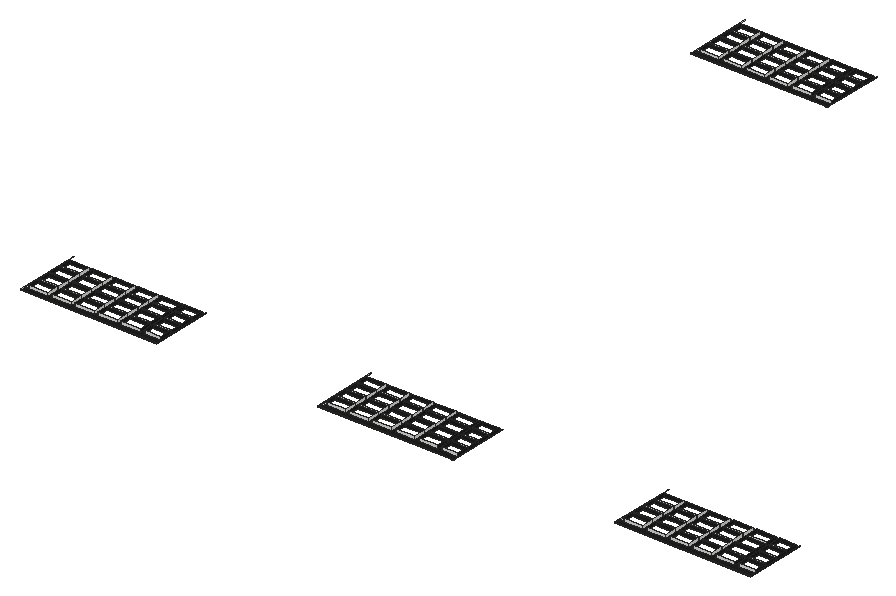
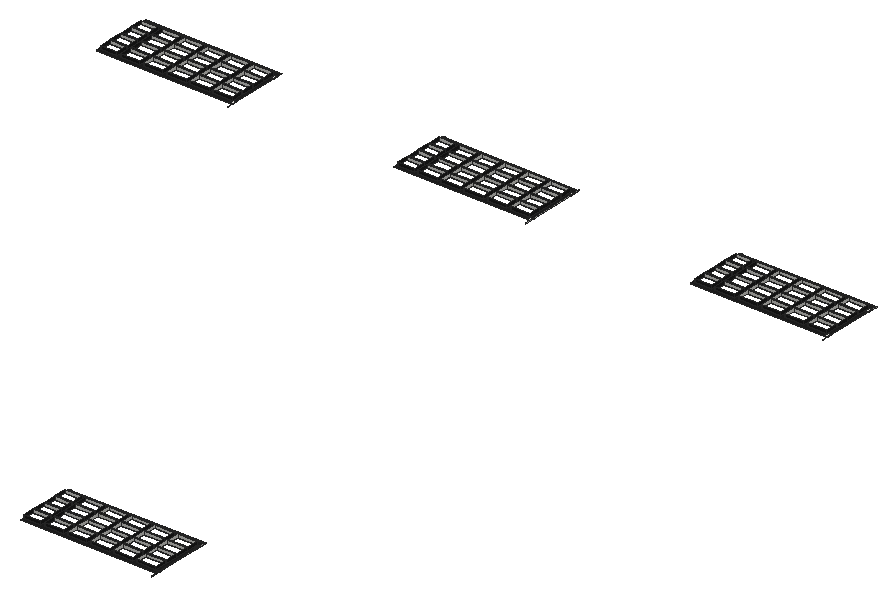
# SketchUp Ruby script. Lengths in inches.
U = 1.inch
M = Sketchup.active_model
def pt(a) = Geom::Point3d.new(a.map { |v| v * U })
def face(e, loops, mat)
  f = e.add_face(loops[0].map { |a| pt(a) })
  loops[1..].each { |l| e.add_face(l.map { |a| pt(a) }).erase! }
  f.material = f.back_material = mat if mat
  f
end
# faces: each face lists its corners as indices into pts; further lists are holes
def faces(e, pts, list, mat = nil) = list.each { |f| face(e, (f[0].is_a?(Array) ? f : [f]).map { |l| l.map { |i| pts[i] } }, mat) }
# xy, xz, yz: faces in a plane at the given z, y or x. An outline is a flat list of corners, or four numbers for a rectangle; further outlines are holes
def ring(l) = l.size == 4 ? [[l[0], l[1]], [l[2], l[1]], [l[2], l[3]], [l[0], l[3]]] : l.each_slice(2).to_a
def flat(e, list, mat, &to3) = list.each { |f| face(e, (f[0].is_a?(Array) ? f : [f]).map { |l| ring(l).map { |u, v| to3.(u, v) } }, mat) }
def xy(e, z, list, mat = nil) = flat(e, list, mat) { |x, y| [x, y, z] }
def xz(e, y, list, mat = nil) = flat(e, list, mat) { |x, z| [x, y, z] }
def yz(e, x, list, mat = nil) = flat(e, list, mat) { |y, z| [x, y, z] }
def lines(e, pts, list) = list.each { |a, b| e.add_line(pt(pts[a]), pt(pts[b])) }
# prism: a flat outline (further loops are holes) pulled along v
def prism(e, loops, v, mat = nil)
  f = face(e, loops, mat); d = Geom::Vector3d.new(v.map { |x| x * U })
  f.pushpull(f.normal.samedirection?(d) ? d.length : -d.length)
end
def box(e, o, s, mat = nil) = prism(e, [[o, [o[0] + s[0], o[1], o[2]], [o[0] + s[0], o[1] + s[1], o[2]], [o[0], o[1] + s[1], o[2]]]], [0, 0, s[2]], mat)
def at(x, y, z, deg = 0) = Geom::Transformation.translation(pt([x, y, z])) * Geom::Transformation.rotation(ORIGIN, Z_AXIS, deg.degrees)
def axes(o, x, y, z) = Geom::Transformation.new([*x, 0, *y, 0, *z, 0, *pt(o).to_a, 1])
def part(name) = M.definitions.add(name)
# library, detail: a bought-in or finely detailed component or shape, given as its bounding box
def library(name, o, s) = part(name).tap { |d| box(d.entities, o, s) }
def detail(e, o, s) = box(e.add_group.entities, o, s)
def put(e, d, t, mat = nil) = e.add_instance(d, t).tap { |i| i.material = mat if mat }
def group(e, t, mat = nil) = e.add_group.tap { |g| g.transformation = t; g.material = mat if mat }.entities
root = M.entities
M.materials.add("[Color M08]").color = [30, 30, 30]
xy(root,115.91,[[264.14,322.4375,270.875,322.71],[1150.61,322.4375,1157.34,322.71],[2037.07,322.4375,2043.8,322.71],[264.14,322.71,270.875,334.4375],[1150.61,322.71,1157.34,334.4375],
  [2037.07,322.71,2043.8,334.4375],[264.14,475.3125,270.875,487.3125],[1150.61,475.3125,1157.34,487.3125],[2037.07,475.3125,2043.8,487.3125],[782.875,2174.43,789.61,2174.7],
  [782.875,2174.7,789.61,2186.43],[782.875,2327.31,789.61,2339.31]])
xy(root,115.91,[[[264.14,305.5,264.14,322.4375,270.875,322.4375,270.875,322.71,275.2,322.71,275.2,334.54,264.14,334.54,264.14,475.3125,275.36,475.3125,275.36,487.3125,671.22,487.3125,671.22,305.5],[412.875,323.5,470.84,323.5,470.84,356.95,412.875,356.95,412.875,362.375,470.84,362.375,470.84,396.41,412.875,396.41,412.875,401.625,470.84,401.625,470.84,435.86,412.875,435.86,412.875,441.875,470.84,441.875,470.84,475.3125,412.875,475.3125,412.875,435.86,401.9375,435.86,401.9375,475.3125,343.98,475.3125,343.98,401.625,401.9375,401.625,401.9375,396.41,343.98,396.41,343.98,362.375,401.9375,362.375,401.9375,435.86,412.875,435.86],[481.77,323.5,539.73,323.5,539.73,396.41,481.77,396.41,481.77,401.625,539.73,401.625,539.73,475.3125,481.77,475.3125,481.77,441.875,539.73,441.875,539.73,435.86,481.77,435.86],[550.67,323.5,608.63,435.86],[275.89,401.625,333.04,435.86],[275.89,362.375,333.04,396.41],[343.98,323.5,401.9375,356.95],[550.67,442.1875,608.63,475.3125],[275.89,323.5,333.04,356.95],[275.89,441.875,333.04,475.3125],[619.57,323.5,669.03,356.95],[619.57,362.95,669.03,396.41],[619.57,402.41,669.03,435.86],[619.57,441.86,669.03,475.3125]],[[1150.61,305.5,1150.61,322.4375,1157.34,322.4375,1157.34,322.71,1161.66,322.71,1161.66,334.54,1150.61,334.54,1150.61,475.3125,1161.82,475.3125,1161.82,487.3125,1557.68,487.3125,1557.68,305.5],[1299.34,323.5,1357.3,323.5,1357.3,356.95,1299.34,356.95,1299.34,362.375,1357.3,362.375,1357.3,396.41,1299.34,396.41,1299.34,401.625,1357.3,401.625,1357.3,435.86,1299.34,435.86,1299.34,441.875,1357.3,441.875,1357.3,475.3125,1299.34,475.3125,1299.34,435.86,1288.4,435.86,1288.4,475.3125,1230.44,475.3125,1230.44,401.625,1288.4,401.625,1288.4,396.41,1230.44,396.41,1230.44,362.375,1288.4,362.375,1288.4,435.86,1299.34,435.86],[1368.24,323.5,1426.2,323.5,1426.2,396.41,1368.24,396.41,1368.24,401.625,1426.2,401.625,1426.2,475.3125,1368.24,475.3125,1368.24,441.875,1426.2,441.875,1426.2,435.86,1368.24,435.86],[1437.14,323.5,1495.1,435.86],[1162.36,401.625,1219.5,435.86],[1162.36,362.375,1219.5,396.41],[1230.44,323.5,1288.4,356.95],[1437.14,442.1875,1495.1,475.3125],[1162.36,323.5,1219.5,356.95],[1162.36,441.875,1219.5,475.3125],[1506.03,323.5,1555.49,356.95],[1506.03,362.95,1555.49,396.41],[1506.03,402.41,1555.49,435.86],[1506.03,441.86,1555.49,475.3125]],[[2037.07,305.5,2037.07,322.4375,2043.8,322.4375,2043.8,322.71,2048.125,322.71,2048.125,334.54,2037.07,334.54,2037.07,475.3125,2048.29,475.3125,2048.29,487.3125,2444.15,487.3125,2444.15,305.5],[2185.8,323.5,2243.76,323.5,2243.76,356.95,2185.8,356.95,2185.8,362.375,2243.76,362.375,2243.76,396.41,2185.8,396.41,2185.8,401.625,2243.76,401.625,2243.76,435.86,2185.8,435.86,2185.8,441.875,2243.76,441.875,2243.76,475.3125,2185.8,475.3125,2185.8,435.86,2174.87,435.86,2174.87,475.3125,2116.91,475.3125,2116.91,401.625,2174.87,401.625,2174.87,396.41,2116.91,396.41,2116.91,362.375,2174.87,362.375,2174.87,435.86,2185.8,435.86],[2254.7,323.5,2312.66,323.5,2312.66,396.41,2254.7,396.41,2254.7,401.625,2312.66,401.625,2312.66,475.3125,2254.7,475.3125,2254.7,441.875,2312.66,441.875,2312.66,435.86,2254.7,435.86],[2323.6,323.5,2381.56,435.86],[2048.82,401.625,2105.97,435.86],[2048.82,362.375,2105.97,396.41],[2116.91,323.5,2174.87,356.95],[2323.6,442.1875,2381.56,475.3125],[2048.82,323.5,2105.97,356.95],[2048.82,441.875,2105.97,475.3125],[2392.5,323.5,2441.96,356.95],[2392.5,362.95,2441.96,396.41],[2392.5,402.41,2441.96,435.86],[2392.5,441.86,2441.96,475.3125]],[270.875,322.71,270.875,334.4375,264.14,334.4375,264.14,334.54,275.2,334.54,275.2,322.71],[1157.34,322.71,1157.34,334.4375,1150.61,334.4375,1150.61,334.54,1161.66,334.54,1161.66,322.71],
  [2043.8,322.71,2043.8,334.4375,2037.07,334.4375,2037.07,334.54,2048.125,334.54,2048.125,322.71],[481.77,356.95,539.73,362.375],[550.67,356.95,608.63,362.875],[1368.24,356.95,1426.2,362.375],[1437.14,356.95,1495.1,362.875],
  [2254.7,356.95,2312.66,362.375],[2323.6,356.95,2381.56,362.875],[550.67,396.41,608.63,401.75],[1437.14,396.41,1495.1,401.75],[2323.6,396.41,2381.56,401.75],
  [343.98,435.86,401.9375,441.875],[1230.44,435.86,1288.4,441.875],[2116.91,435.86,2174.87,441.875],[270.875,475.3125,275.36,487.3125],[1157.34,475.3125,1161.82,487.3125],
  [2043.8,475.3125,2048.29,487.3125],[[782.875,2157.49,782.875,2174.43,789.61,2174.43,789.61,2174.7,793.93,2174.7,793.93,2186.53,782.875,2186.53,782.875,2327.31,794.09,2327.31,794.09,2339.31,1189.95,2339.31,1189.95,2157.49],[931.61,2175.49,989.57,2175.49,989.57,2208.95,931.61,2208.95,931.61,2214.37,989.57,2214.37,989.57,2248.4,931.61,2248.4,931.61,2253.62,989.57,2253.62,989.57,2287.85,931.61,2287.85,931.61,2293.87,989.57,2293.87,989.57,2327.31,931.61,2327.31,931.61,2287.85,920.67,2287.85,920.67,2327.31,862.71,2327.31,862.71,2253.62,920.67,2253.62,920.67,2248.4,862.71,2248.4,862.71,2214.37,920.67,2214.37,920.67,2287.85,931.61,2287.85],[1000.51,2175.49,1058.47,2175.49,1058.47,2248.4,1000.51,2248.4,1000.51,2253.62,1058.47,2253.62,1058.47,2327.31,1000.51,2327.31,1000.51,2293.87,1058.47,2293.87,1058.47,2287.85,1000.51,2287.85],[1069.4,2175.49,1127.36,2287.85],[794.625,2253.62,851.77,2287.85],[794.625,2214.37,851.77,2248.4],[862.71,2175.49,920.67,2208.95],[1069.4,2294.18,1127.36,2327.31],[794.625,2175.49,851.77,2208.95],[794.625,2293.87,851.77,2327.31],[1138.3,2293.85,1187.76,2327.31],[1138.3,2175.49,1187.76,2208.95],[1138.3,2214.95,1187.76,2248.4],[1138.3,2254.4,1187.76,2287.85]],[789.61,2174.7,789.61,2186.43,782.875,2186.43,782.875,2186.53,793.93,2186.53,793.93,2174.7],[1000.51,2208.95,1058.47,2214.37],[1069.4,2208.95,1127.36,2214.87],
  [1069.4,2248.4,1127.36,2253.74],[862.71,2287.85,920.67,2293.87],[789.61,2327.31,794.09,2339.31]],"[Color M08]")
xz(root,305.5,[[264.14,115.91,671.22,117.06],[1150.61,115.91,1557.68,117.06],[2037.07,115.91,2444.15,117.06]],"[Color M08]")
xz(root,323.5,[[275.89,115.91,333.04,125.0625],[343.98,115.91,401.9375,125.0625],[412.875,115.91,470.84,125.0625],[481.77,115.91,539.73,125.0625],[550.67,115.91,608.63,125.0625],
  [619.57,115.91,669.03,125.0625],[1162.36,115.91,1219.5,125.0625],[1230.44,115.91,1288.4,125.0625],[1299.34,115.91,1357.3,125.0625],[1368.24,115.91,1426.2,125.0625],
  [1437.14,115.91,1495.1,125.0625],[1506.03,115.91,1555.49,125.0625],[2048.82,115.91,2105.97,125.0625],[2116.91,115.91,2174.87,125.0625],[2185.8,115.91,2243.76,125.0625],
  [2254.7,115.91,2312.66,125.0625],[2323.6,115.91,2381.56,125.0625],[2392.5,115.91,2441.96,125.0625]])
xz(root,356.95,[[275.89,115.91,333.04,125.0625],[343.98,115.91,401.9375,125.0625],[412.875,115.91,470.84,125.0625],[481.77,115.91,539.73,125.0625],[550.67,115.91,608.63,125.0625],
  [619.57,115.91,669.03,125.0625],[1162.36,115.91,1219.5,125.0625],[1230.44,115.91,1288.4,125.0625],[1299.34,115.91,1357.3,125.0625],[1368.24,115.91,1426.2,125.0625],
  [1437.14,115.91,1495.1,125.0625],[1506.03,115.91,1555.49,125.0625],[2048.82,115.91,2105.97,125.0625],[2116.91,115.91,2174.87,125.0625],[2185.8,115.91,2243.76,125.0625],
  [2254.7,115.91,2312.66,125.0625],[2323.6,115.91,2381.56,125.0625],[2392.5,115.91,2441.96,125.0625]],"[Color M08]")
xz(root,362.375,[[275.89,115.91,333.04,125.0625],[343.98,115.91,401.9375,125.0625],[412.875,115.91,470.84,125.0625],[481.77,115.91,539.73,125.0625],[1162.36,115.91,1219.5,125.0625],
  [1230.44,115.91,1288.4,125.0625],[1299.34,115.91,1357.3,125.0625],[1368.24,115.91,1426.2,125.0625],[2048.82,115.91,2105.97,125.0625],[2116.91,115.91,2174.87,125.0625],
  [2185.8,115.91,2243.76,125.0625],[2254.7,115.91,2312.66,125.0625]])
xz(root,362.875,[[550.67,115.91,608.63,125.0625],[1437.14,115.91,1495.1,125.0625],[2323.6,115.91,2381.56,125.0625]])
xz(root,362.95,[[619.57,115.91,669.03,125.0625],[1506.03,115.91,1555.49,125.0625],[2392.5,115.91,2441.96,125.0625]])
xz(root,396.41,[[275.89,115.91,333.04,125.0625],[343.98,115.91,401.9375,125.0625],[412.875,115.91,470.84,125.0625],[481.77,115.91,539.73,125.0625],[550.67,115.91,608.63,125.0625],
  [619.57,115.91,669.03,125.0625],[1162.36,115.91,1219.5,125.0625],[1230.44,115.91,1288.4,125.0625],[1299.34,115.91,1357.3,125.0625],[1368.24,115.91,1426.2,125.0625],
  [1437.14,115.91,1495.1,125.0625],[1506.03,115.91,1555.49,125.0625],[2048.82,115.91,2105.97,125.0625],[2116.91,115.91,2174.87,125.0625],[2185.8,115.91,2243.76,125.0625],
  [2254.7,115.91,2312.66,125.0625],[2323.6,115.91,2381.56,125.0625],[2392.5,115.91,2441.96,125.0625]],"[Color M08]")
xz(root,401.625,[[275.89,115.91,333.04,125.0625],[343.98,115.91,401.9375,125.0625],[412.875,115.91,470.84,125.0625],[481.77,115.91,539.73,125.0625],[1162.36,115.91,1219.5,125.0625],
  [1230.44,115.91,1288.4,125.0625],[1299.34,115.91,1357.3,125.0625],[1368.24,115.91,1426.2,125.0625],[2048.82,115.91,2105.97,125.0625],[2116.91,115.91,2174.87,125.0625],
  [2185.8,115.91,2243.76,125.0625],[2254.7,115.91,2312.66,125.0625]])
xz(root,401.75,[[550.67,115.91,608.63,125.0625],[1437.14,115.91,1495.1,125.0625],[2323.6,115.91,2381.56,125.0625]])
xz(root,402.41,[[619.57,115.91,669.03,125.0625],[1506.03,115.91,1555.49,125.0625],[2392.5,115.91,2441.96,125.0625]])
xz(root,435.86,[[275.89,115.91,333.04,125.0625],[343.98,115.91,401.9375,125.0625],[412.875,115.91,470.84,125.0625],[481.77,115.91,539.73,125.0625],[550.67,115.91,608.63,125.0625],
  [619.57,115.91,669.03,125.0625],[1162.36,115.91,1219.5,125.0625],[1230.44,115.91,1288.4,125.0625],[1299.34,115.91,1357.3,125.0625],[1368.24,115.91,1426.2,125.0625],
  [1437.14,115.91,1495.1,125.0625],[1506.03,115.91,1555.49,125.0625],[2048.82,115.91,2105.97,125.0625],[2116.91,115.91,2174.87,125.0625],[2185.8,115.91,2243.76,125.0625],
  [2254.7,115.91,2312.66,125.0625],[2323.6,115.91,2381.56,125.0625],[2392.5,115.91,2441.96,125.0625]],"[Color M08]")
xz(root,441.86,[[619.57,115.91,669.03,125.0625],[1506.03,115.91,1555.49,125.0625],[2392.5,115.91,2441.96,125.0625]])
xz(root,441.875,[[275.89,115.91,333.04,125.0625],[343.98,115.91,401.9375,125.0625],[412.875,115.91,470.84,125.0625],[481.77,115.91,539.73,125.0625],[1162.36,115.91,1219.5,125.0625],
  [1230.44,115.91,1288.4,125.0625],[1299.34,115.91,1357.3,125.0625],[1368.24,115.91,1426.2,125.0625],[2048.82,115.91,2105.97,125.0625],[2116.91,115.91,2174.87,125.0625],
  [2185.8,115.91,2243.76,125.0625],[2254.7,115.91,2312.66,125.0625]])
xz(root,442.1875,[[550.67,115.91,608.63,125.0625],[1437.14,115.91,1495.1,125.0625],[2323.6,115.91,2381.56,125.0625]])
xz(root,475.3125,[[275.89,115.91,333.04,125.0625],[343.98,115.91,401.9375,125.0625],[412.875,115.91,470.84,125.0625],[481.77,115.91,539.73,125.0625],[550.67,115.91,608.63,125.0625],
  [619.57,115.91,669.03,125.0625],[1162.36,115.91,1219.5,125.0625],[1230.44,115.91,1288.4,125.0625],[1299.34,115.91,1357.3,125.0625],[1368.24,115.91,1426.2,125.0625],
  [1437.14,115.91,1495.1,125.0625],[1506.03,115.91,1555.49,125.0625],[2048.82,115.91,2105.97,125.0625],[2116.91,115.91,2174.87,125.0625],[2185.8,115.91,2243.76,125.0625],
  [2254.7,115.91,2312.66,125.0625],[2323.6,115.91,2381.56,125.0625],[2392.5,115.91,2441.96,125.0625]],"[Color M08]")
xz(root,2157.49,[[782.875,115.91,1189.95,117.06]],"[Color M08]")
xz(root,2175.49,[[794.625,115.91,851.77,125.0625],[862.71,115.91,920.67,125.0625],[931.61,115.91,989.57,125.0625],[1000.51,115.91,1058.47,125.0625],[1069.4,115.91,1127.36,125.0625],
  [1138.3,115.91,1187.76,125.0625]])
xz(root,2208.95,[[794.625,115.91,851.77,125.0625],[862.71,115.91,920.67,125.0625],[931.61,115.91,989.57,125.0625],[1000.51,115.91,1058.47,125.0625],[1069.4,115.91,1127.36,125.0625],
  [1138.3,115.91,1187.76,125.0625]],"[Color M08]")
xz(root,2214.37,[[794.625,115.91,851.77,125.0625],[862.71,115.91,920.67,125.0625],[931.61,115.91,989.57,125.0625],[1000.51,115.91,1058.47,125.0625]])
xz(root,2214.87,[[1069.4,115.91,1127.36,125.0625]])
xz(root,2214.95,[[1138.3,115.91,1187.76,125.0625]])
xz(root,2248.4,[[794.625,115.91,851.77,125.0625],[862.71,115.91,920.67,125.0625],[931.61,115.91,989.57,125.0625],[1000.51,115.91,1058.47,125.0625],[1069.4,115.91,1127.36,125.0625],
  [1138.3,115.91,1187.76,125.0625]],"[Color M08]")
xz(root,2253.62,[[794.625,115.91,851.77,125.0625],[862.71,115.91,920.67,125.0625],[931.61,115.91,989.57,125.0625],[1000.51,115.91,1058.47,125.0625]])
xz(root,2253.74,[[1069.4,115.91,1127.36,125.0625]])
xz(root,2254.4,[[1138.3,115.91,1187.76,125.0625]])
xz(root,2287.85,[[794.625,115.91,851.77,125.0625],[862.71,115.91,920.67,125.0625],[931.61,115.91,989.57,125.0625],[1000.51,115.91,1058.47,125.0625],[1069.4,115.91,1127.36,125.0625],
  [1138.3,115.91,1187.76,125.0625]],"[Color M08]")
xz(root,2293.85,[[1138.3,115.91,1187.76,125.0625]])
xz(root,2293.87,[[794.625,115.91,851.77,125.0625],[862.71,115.91,920.67,125.0625],[931.61,115.91,989.57,125.0625],[1000.51,115.91,1058.47,125.0625]])
xz(root,2294.18,[[1069.4,115.91,1127.36,125.0625]])
xz(root,2327.31,[[794.625,115.91,851.77,125.0625],[862.71,115.91,920.67,125.0625],[931.61,115.91,989.57,125.0625],[1000.51,115.91,1058.47,125.0625],[1069.4,115.91,1127.36,125.0625],
  [1138.3,115.91,1187.76,125.0625]],"[Color M08]")
yz(root,264.14,[[305.5,115.66,322.71,115.91],[322.71,115.66,334.4375,115.91],[334.4375,115.66,475.3125,115.91],[475.3125,115.66,487.3125,115.91],[305.5,115.91,305.5,117.06,306.625,117.06,306.625,117.65,505.3125,117.65,505.3125,115.91]])
yz(root,264.14,[[487.3125,115.66,505.3125,115.91]],"[Color M08]")
yz(root,275.89,[[323.5,115.91,356.95,125.0625],[362.375,115.91,396.41,125.0625],[401.625,115.91,435.86,125.0625],[441.875,115.91,475.3125,125.0625]],"[Color M08]")
yz(root,333.04,[[323.5,115.91,356.95,125.0625],[362.375,115.91,396.41,125.0625],[401.625,115.91,435.86,125.0625],[441.875,115.91,475.3125,125.0625]])
yz(root,343.98,[[323.5,115.91,356.95,125.0625],[362.375,115.91,396.41,125.0625],[401.625,115.91,435.86,125.0625],[441.875,115.91,475.3125,125.0625]],"[Color M08]")
yz(root,401.9375,[[323.5,115.91,356.95,125.0625],[362.375,115.91,396.41,125.0625],[401.625,115.91,435.86,125.0625],[441.875,115.91,475.3125,125.0625]])
yz(root,412.875,[[323.5,115.91,356.95,125.0625],[362.375,115.91,396.41,125.0625],[401.625,115.91,435.86,125.0625],[441.875,115.91,475.3125,125.0625]],"[Color M08]")
yz(root,470.84,[[323.5,115.91,356.95,125.0625],[362.375,115.91,396.41,125.0625],[401.625,115.91,435.86,125.0625],[441.875,115.91,475.3125,125.0625]])
yz(root,481.77,[[323.5,115.91,356.95,125.0625],[362.375,115.91,396.41,125.0625],[401.625,115.91,435.86,125.0625],[441.875,115.91,475.3125,125.0625]],"[Color M08]")
yz(root,539.73,[[323.5,115.91,356.95,125.0625],[362.375,115.91,396.41,125.0625],[401.625,115.91,435.86,125.0625],[441.875,115.91,475.3125,125.0625]])
yz(root,550.67,[[323.5,115.91,356.95,125.0625],[362.875,115.91,396.41,125.0625],[401.75,115.91,435.86,125.0625],[442.1875,115.91,475.3125,125.0625]],"[Color M08]")
yz(root,608.63,[[323.5,115.91,356.95,125.0625],[362.875,115.91,396.41,125.0625],[401.75,115.91,435.86,125.0625],[442.1875,115.91,475.3125,125.0625]],"[Color M08]")
yz(root,619.57,[[323.5,115.91,356.95,125.0625],[362.95,115.91,396.41,125.0625],[402.41,115.91,435.86,125.0625],[441.86,115.91,475.3125,125.0625]],"[Color M08]")
yz(root,669.03,[[323.5,115.91,356.95,125.0625],[362.95,115.91,396.41,125.0625],[402.41,115.91,435.86,125.0625],[441.86,115.91,475.3125,125.0625]],"[Color M08]")
yz(root,671.22,[[305.5,115.91,487.3125,117.06]],"[Color M08]")
yz(root,782.875,[[2157.49,115.66,2174.7,115.91],[2174.7,115.66,2186.43,115.91],[2186.43,115.66,2327.31,115.91],[2327.31,115.66,2339.31,115.91],[2157.49,115.91,2157.49,117.06,2158.62,117.06,2158.62,117.65,2357.31,117.65,2357.31,115.91]])
yz(root,782.875,[[2339.31,115.66,2357.31,115.91]],"[Color M08]")
yz(root,794.625,[[2175.49,115.91,2208.95,125.0625],[2214.37,115.91,2248.4,125.0625],[2253.62,115.91,2287.85,125.0625],[2293.87,115.91,2327.31,125.0625]],"[Color M08]")
yz(root,851.77,[[2175.49,115.91,2208.95,125.0625],[2214.37,115.91,2248.4,125.0625],[2253.62,115.91,2287.85,125.0625],[2293.87,115.91,2327.31,125.0625]])
yz(root,862.71,[[2175.49,115.91,2208.95,125.0625],[2214.37,115.91,2248.4,125.0625],[2253.62,115.91,2287.85,125.0625],[2293.87,115.91,2327.31,125.0625]],"[Color M08]")
yz(root,920.67,[[2175.49,115.91,2208.95,125.0625],[2214.37,115.91,2248.4,125.0625],[2253.62,115.91,2287.85,125.0625],[2293.87,115.91,2327.31,125.0625]])
yz(root,931.61,[[2175.49,115.91,2208.95,125.0625],[2214.37,115.91,2248.4,125.0625],[2253.62,115.91,2287.85,125.0625],[2293.87,115.91,2327.31,125.0625]],"[Color M08]")
yz(root,989.57,[[2175.49,115.91,2208.95,125.0625],[2214.37,115.91,2248.4,125.0625],[2253.62,115.91,2287.85,125.0625],[2293.87,115.91,2327.31,125.0625]])
yz(root,1000.51,[[2175.49,115.91,2208.95,125.0625],[2214.37,115.91,2248.4,125.0625],[2253.62,115.91,2287.85,125.0625],[2293.87,115.91,2327.31,125.0625]],"[Color M08]")
yz(root,1058.47,[[2175.49,115.91,2208.95,125.0625],[2214.37,115.91,2248.4,125.0625],[2253.62,115.91,2287.85,125.0625],[2293.87,115.91,2327.31,125.0625]])
yz(root,1069.4,[[2175.49,115.91,2208.95,125.0625],[2214.87,115.91,2248.4,125.0625],[2253.74,115.91,2287.85,125.0625],[2294.18,115.91,2327.31,125.0625]],"[Color M08]")
yz(root,1127.36,[[2175.49,115.91,2208.95,125.0625],[2214.87,115.91,2248.4,125.0625],[2253.74,115.91,2287.85,125.0625],[2294.18,115.91,2327.31,125.0625]],"[Color M08]")
yz(root,1138.3,[[2175.49,115.91,2208.95,125.0625],[2214.95,115.91,2248.4,125.0625],[2254.4,115.91,2287.85,125.0625],[2293.85,115.91,2327.31,125.0625]],"[Color M08]")
yz(root,1150.61,[[305.5,115.66,322.71,115.91],[322.71,115.66,334.4375,115.91],[334.4375,115.66,475.3125,115.91],[475.3125,115.66,487.3125,115.91],[305.5,115.91,305.5,117.06,306.625,117.06,306.625,117.65,505.3125,117.65,505.3125,115.91]])
yz(root,1150.61,[[487.3125,115.66,505.3125,115.91]],"[Color M08]")
yz(root,1162.36,[[323.5,115.91,356.95,125.0625],[362.375,115.91,396.41,125.0625],[401.625,115.91,435.86,125.0625],[441.875,115.91,475.3125,125.0625]],"[Color M08]")
yz(root,1187.76,[[2175.49,115.91,2208.95,125.0625],[2214.95,115.91,2248.4,125.0625],[2254.4,115.91,2287.85,125.0625],[2293.85,115.91,2327.31,125.0625]],"[Color M08]")
yz(root,1189.95,[[2157.49,115.91,2339.31,117.06]],"[Color M08]")
yz(root,1219.5,[[323.5,115.91,356.95,125.0625],[362.375,115.91,396.41,125.0625],[401.625,115.91,435.86,125.0625],[441.875,115.91,475.3125,125.0625]])
yz(root,1230.44,[[323.5,115.91,356.95,125.0625],[362.375,115.91,396.41,125.0625],[401.625,115.91,435.86,125.0625],[441.875,115.91,475.3125,125.0625]],"[Color M08]")
yz(root,1288.4,[[323.5,115.91,356.95,125.0625],[362.375,115.91,396.41,125.0625],[401.625,115.91,435.86,125.0625],[441.875,115.91,475.3125,125.0625]])
yz(root,1299.34,[[323.5,115.91,356.95,125.0625],[362.375,115.91,396.41,125.0625],[401.625,115.91,435.86,125.0625],[441.875,115.91,475.3125,125.0625]],"[Color M08]")
yz(root,1357.3,[[323.5,115.91,356.95,125.0625],[362.375,115.91,396.41,125.0625],[401.625,115.91,435.86,125.0625],[441.875,115.91,475.3125,125.0625]])
yz(root,1368.24,[[323.5,115.91,356.95,125.0625],[362.375,115.91,396.41,125.0625],[401.625,115.91,435.86,125.0625],[441.875,115.91,475.3125,125.0625]],"[Color M08]")
yz(root,1426.2,[[323.5,115.91,356.95,125.0625],[362.375,115.91,396.41,125.0625],[401.625,115.91,435.86,125.0625],[441.875,115.91,475.3125,125.0625]])
yz(root,1437.14,[[323.5,115.91,356.95,125.0625],[362.875,115.91,396.41,125.0625],[401.75,115.91,435.86,125.0625],[442.1875,115.91,475.3125,125.0625]],"[Color M08]")
yz(root,1495.1,[[323.5,115.91,356.95,125.0625],[362.875,115.91,396.41,125.0625],[401.75,115.91,435.86,125.0625],[442.1875,115.91,475.3125,125.0625]],"[Color M08]")
yz(root,1506.03,[[323.5,115.91,356.95,125.0625],[362.95,115.91,396.41,125.0625],[402.41,115.91,435.86,125.0625],[441.86,115.91,475.3125,125.0625]],"[Color M08]")
yz(root,1555.49,[[323.5,115.91,356.95,125.0625],[362.95,115.91,396.41,125.0625],[402.41,115.91,435.86,125.0625],[441.86,115.91,475.3125,125.0625]],"[Color M08]")
yz(root,1557.68,[[305.5,115.91,487.3125,117.06]],"[Color M08]")
yz(root,2037.07,[[305.5,115.66,322.71,115.91],[322.71,115.66,334.4375,115.91],[334.4375,115.66,475.3125,115.91],[475.3125,115.66,487.3125,115.91],[305.5,115.91,305.5,117.06,306.625,117.06,306.625,117.65,505.3125,117.65,505.3125,115.91]])
yz(root,2037.07,[[487.3125,115.66,505.3125,115.91]],"[Color M08]")
yz(root,2048.82,[[323.5,115.91,356.95,125.0625],[362.375,115.91,396.41,125.0625],[401.625,115.91,435.86,125.0625],[441.875,115.91,475.3125,125.0625]],"[Color M08]")
yz(root,2105.97,[[323.5,115.91,356.95,125.0625],[362.375,115.91,396.41,125.0625],[401.625,115.91,435.86,125.0625],[441.875,115.91,475.3125,125.0625]])
yz(root,2116.91,[[323.5,115.91,356.95,125.0625],[362.375,115.91,396.41,125.0625],[401.625,115.91,435.86,125.0625],[441.875,115.91,475.3125,125.0625]],"[Color M08]")
yz(root,2174.87,[[323.5,115.91,356.95,125.0625],[362.375,115.91,396.41,125.0625],[401.625,115.91,435.86,125.0625],[441.875,115.91,475.3125,125.0625]])
yz(root,2185.8,[[323.5,115.91,356.95,125.0625],[362.375,115.91,396.41,125.0625],[401.625,115.91,435.86,125.0625],[441.875,115.91,475.3125,125.0625]],"[Color M08]")
yz(root,2243.76,[[323.5,115.91,356.95,125.0625],[362.375,115.91,396.41,125.0625],[401.625,115.91,435.86,125.0625],[441.875,115.91,475.3125,125.0625]])
yz(root,2254.7,[[323.5,115.91,356.95,125.0625],[362.375,115.91,396.41,125.0625],[401.625,115.91,435.86,125.0625],[441.875,115.91,475.3125,125.0625]],"[Color M08]")
yz(root,2312.66,[[323.5,115.91,356.95,125.0625],[362.375,115.91,396.41,125.0625],[401.625,115.91,435.86,125.0625],[441.875,115.91,475.3125,125.0625]])
yz(root,2323.6,[[323.5,115.91,356.95,125.0625],[362.875,115.91,396.41,125.0625],[401.75,115.91,435.86,125.0625],[442.1875,115.91,475.3125,125.0625]],"[Color M08]")
yz(root,2381.56,[[323.5,115.91,356.95,125.0625],[362.875,115.91,396.41,125.0625],[401.75,115.91,435.86,125.0625],[442.1875,115.91,475.3125,125.0625]],"[Color M08]")
yz(root,2392.5,[[323.5,115.91,356.95,125.0625],[362.95,115.91,396.41,125.0625],[402.41,115.91,435.86,125.0625],[441.86,115.91,475.3125,125.0625]],"[Color M08]")
yz(root,2441.96,[[323.5,115.91,356.95,125.0625],[362.95,115.91,396.41,125.0625],[402.41,115.91,435.86,125.0625],[441.86,115.91,475.3125,125.0625]],"[Color M08]")
yz(root,2444.15,[[305.5,115.91,487.3125,117.06]],"[Color M08]")
